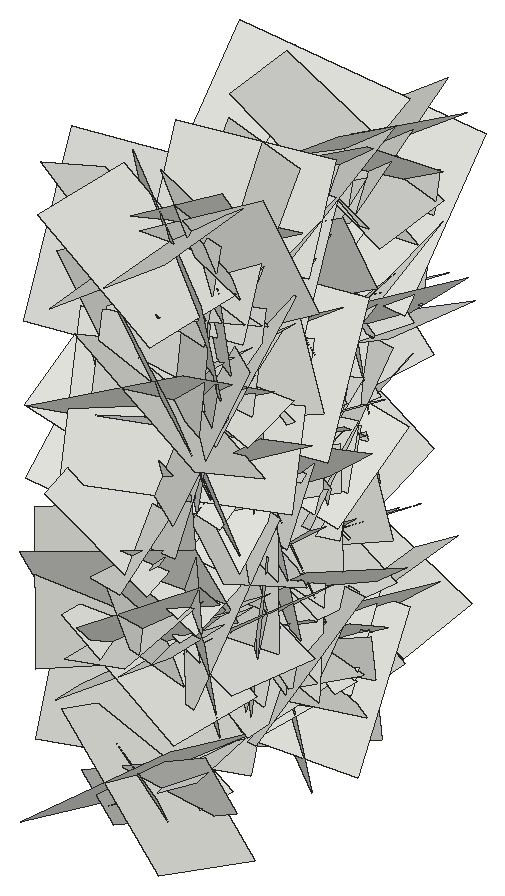
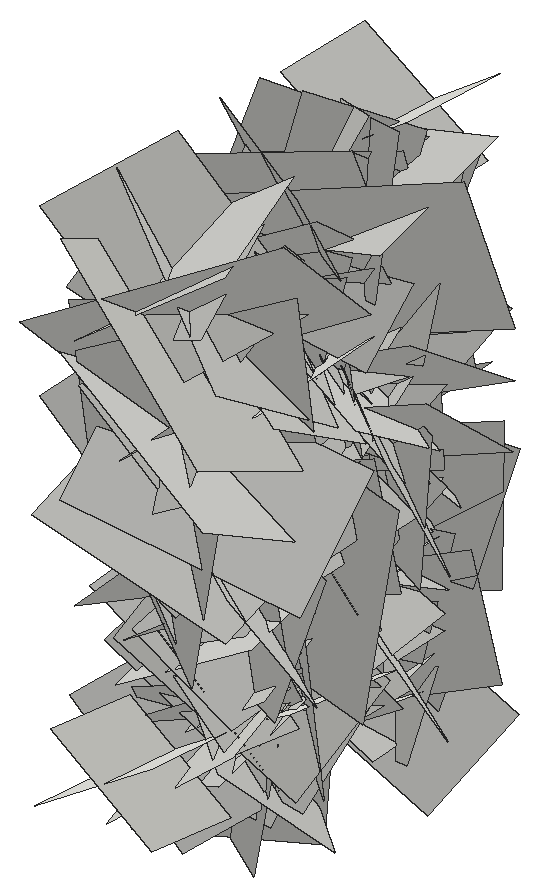
# SketchUp Ruby script. Lengths in inches.
U = 1.inch
M = Sketchup.active_model
def pt(a) = Geom::Point3d.new(a.map { |v| v * U })
def face(e, loops, mat)
  f = e.add_face(loops[0].map { |a| pt(a) })
  loops[1..].each { |l| e.add_face(l.map { |a| pt(a) }).erase! }
  f.material = f.back_material = mat if mat
  f
end
# faces: each face lists its corners as indices into pts; further lists are holes
def faces(e, pts, list, mat = nil) = list.each { |f| face(e, (f[0].is_a?(Array) ? f : [f]).map { |l| l.map { |i| pts[i] } }, mat) }
# xy, xz, yz: faces in a plane at the given z, y or x. An outline is a flat list of corners, or four numbers for a rectangle; further outlines are holes
def ring(l) = l.size == 4 ? [[l[0], l[1]], [l[2], l[1]], [l[2], l[3]], [l[0], l[3]]] : l.each_slice(2).to_a
def flat(e, list, mat, &to3) = list.each { |f| face(e, (f[0].is_a?(Array) ? f : [f]).map { |l| ring(l).map { |u, v| to3.(u, v) } }, mat) }
def xy(e, z, list, mat = nil) = flat(e, list, mat) { |x, y| [x, y, z] }
def xz(e, y, list, mat = nil) = flat(e, list, mat) { |x, z| [x, y, z] }
def yz(e, x, list, mat = nil) = flat(e, list, mat) { |y, z| [x, y, z] }
def lines(e, pts, list) = list.each { |a, b| e.add_line(pt(pts[a]), pt(pts[b])) }
# prism: a flat outline (further loops are holes) pulled along v
def prism(e, loops, v, mat = nil)
  f = face(e, loops, mat); d = Geom::Vector3d.new(v.map { |x| x * U })
  f.pushpull(f.normal.samedirection?(d) ? d.length : -d.length)
end
def box(e, o, s, mat = nil) = prism(e, [[o, [o[0] + s[0], o[1], o[2]], [o[0] + s[0], o[1] + s[1], o[2]], [o[0], o[1] + s[1], o[2]]]], [0, 0, s[2]], mat)
def at(x, y, z, deg = 0) = Geom::Transformation.translation(pt([x, y, z])) * Geom::Transformation.rotation(ORIGIN, Z_AXIS, deg.degrees)
def axes(o, x, y, z) = Geom::Transformation.new([*x, 0, *y, 0, *z, 0, *pt(o).to_a, 1])
def part(name) = M.definitions.add(name)
# library, detail: a bought-in or finely detailed component or shape, given as its bounding box
def library(name, o, s) = part(name).tap { |d| box(d.entities, o, s) }
def detail(e, o, s) = box(e.add_group.entities, o, s)
def put(e, d, t, mat = nil) = e.add_instance(d, t).tap { |i| i.material = mat if mat }
def group(e, t, mat = nil) = e.add_group.tap { |g| g.transformation = t; g.material = mat if mat }.entities
root = M.entities
c1 = part("Component\#6")
p = [[0.01,0,0],[0,3.24,4.54],[4.32,3.24,4.54],[4.33,0,0]]
faces(c1.entities,p,[[0,1,2,3]])
put(root,c1,axes([18.5,190.14,35.27],[-0.30668,1.10496,-0.445],[-0.14325,-0.48543,-1.11748],[-1.25452,-0.21469,0.23639]))
put(root,c1,axes([18.5,186.51,25.44],[0.00901,-0.3677,1.34811],[-0.26845,1.32541,0.3631],[-1.45667,-0.24653,-0.05858]))
put(root,c1,axes([18.5,188.1875,39.24],[-0.00053,-0.50504,-1.25708],[-0.1621,-1.24903,0.50186],[-1.42684,0.14209,-0.05655]))
put(root,c1,axes([18.5,180.73,30.67],[-0.05707,0.69485,1.12415],[0.04583,1.1254,-0.69356],[-1.4001,0.00851,-0.06852]))
put(root,c1,axes([18.5,188.72,38.18],[-0.108,1.17484,0.54266],[0.09899,0.5496,-1.17232],[-1.36819,-0.05298,-0.12766]))
put(root,c1,axes([18.5,187.26,33.24],[-0.066,-0.95024,-0.64083],[-0.19237,-0.6255,0.94515],[-1.19957,0.15259,-0.11631]))
put(root,c1,axes([18.5,181.61,25.33],[0.14764,0.72138,1.18272],[-0.09804,1.19088,-0.71546],[-1.46521,-0.007,0.16705]))
put(root,c1,axes([18.5,184.99,36.41],[-0.13687,-0.99381,0.45239],[-0.15227,0.46704,0.985],[-1.14738,0.05657,-0.18469]))
put(root,c1,axes([18.5,190.5,33.59],[-0.11278,1.05886,-0.21225],[-0.21462,-0.22906,-1.04119],[-1.12442,-0.06248,0.22002]))
put(root,c1,axes([18.5,187.29,32.09],[0.03087,-0.89426,-0.74249],[-0.26998,-0.72958,0.86873],[-1.20212,0.14089,-0.21417]))
put(root,c1,axes([18.5,186.91,28.91],[0.08475,0.77289,1.06783],[-0.0494,1.07079,-0.77154],[-1.39641,0.00903,0.0921]))
put(root,c1,axes([18.5,188.57,34.3],[0.02784,1.05016,0.5271],[-0.1514,0.52617,-1.0412],[-1.23628,-0.04079,0.13938]))
put(root,c1,axes([18.5,194.96,38.36],[0.08597,-0.96025,-0.92678],[0.03419,-0.92681,0.9631],[-1.41421,-0.08078,-0.03305]))
put(root,c1,axes([18.5,185.59,36.56],[-0.07365,1.00309,0.56692],[-0.00038,0.56794,-1.00493],[-1.22135,-0.06067,-0.03387]))
put(root,c1,axes([18.5,190.1,29],[-0.15352,-0.05709,1.12322],[0.06907,1.13017,0.06585],[-1.19015,0.07295,-0.14107]))
put(root,c1,axes([18.5,182.88,33.98],[-0.05541,0.90127,0.55592],[-0.17138,0.54328,-0.89597],[-1.1093,-0.12895,0.11065]))
put(root,c1,axes([18.5,181.98,27.65],[-0.03848,-0.07343,1.06513],[-0.13392,1.05855,0.06867],[-1.12376,-0.12364,-0.04466]))
put(root,c1,axes([14.53,188.74,27.6],[-0.13014,-0.45431,-0.37588],[-0.00674,-0.3829,0.46487],[0.62498,-0.09873,-0.07326]))
put(root,c1,axes([18.5,192.86,38.11],[-0.10772,-0.0541,-1.0459],[-0.04447,-1.04976,0.05837],[-1.10925,0.04734,0.09923]))
put(root,c1,axes([18.5,187.65,25.55],[-0.14301,-0.32766,0.90945],[-0.11586,0.91755,0.31436],[-1.01811,-0.05839,-0.16352]))
put(root,c1,axes([14.53,191.07,24.72],[-0.08022,-0.60182,-0.03468],[-0.03515,-0.03074,0.60586],[0.63802,-0.07736,0.02902]))
put(root,c1,axes([18.5,189.26,31.29],[-0.07003,-0.18149,-1.00879],[-0.05402,-1.00905,0.18487],[-1.08514,0.06195,0.0559]))
put(root,c1,axes([18.5,184.16,23.6],[-0.00632,0.19994,1.20323],[0.15077,1.19515,-0.1979],[-1.28409,0.13934,-0.02916]))
put(root,c1,axes([14.53,183.51,30.36],[-0.10644,-0.42009,-0.4575],[0.01901,-0.46521,0.42323],[0.65811,-0.0545,-0.08622]))
put(root,c1,axes([14.53,191.45,35.51],[-0.13227,0.51495,-0.41011],[-0.00116,-0.41758,-0.52399],[0.6978,0.09692,-0.07861]))
put(root,c1,axes([18.5,186.92,28.87],[-0.11772,1.08189,-0.3436],[0.18933,-0.32428,-1.0788],[-1.18826,-0.15885,-0.13785]))
put(root,c1,axes([18.5,185.29,39.56],[-0.11827,0.82487,-0.51088],[-0.03346,-0.51706,-0.82795],[-1.02793,-0.07808,0.08573]))
put(root,c1,axes([14.53,188.83,29.07],[-0.04972,0.59189,0.16701],[-0.02122,0.16593,-0.59371],[0.65156,0.05057,-0.00659]))
put(root,c1,axes([18.5,190.19,31.82],[-0.07854,-1.04848,0.11995],[0.05802,0.11627,1.05008],[-1.11713,0.07975,0.0461]))
put(root,c1,axes([14.53,186.02,29.02],[-0.12909,0.32312,-0.64935],[-0.06195,-0.66067,-0.31779],[0.76632,0.00102,-0.13508]))
put(root,c1,axes([18.5,185.55,26.35],[-0.05433,-0.24183,-1.04679],[0.06418,-1.04696,0.23891],[-1.13701,-0.04754,0.0635]))
put(root,c1,axes([18.5,185.63,37.94],[0.10296,1.07287,0.66666],[0.13207,0.65722,-1.07584],[-1.33238,0.14805,-0.05512]))
put(root,c1,axes([18.5,189.07,22.99],[-0.09993,-0.91741,-0.05408],[-0.10319,-0.04408,0.91762],[-0.96866,0.09934,-0.09218]))
put(root,c1,axes([14.53,193.29,29.97],[0.02765,-0.60791,0.13872],[-0.08921,0.13414,0.60366],[0.6549,0.04394,0.07638]))
put(root,c1,axes([14.53,188.93,38.32],[-0.06934,0.59373,0.25],[0.00198,0.25145,-0.59671],[0.68287,0.05956,0.02711]))
put(root,c1,axes([14.53,179.78,31.84],[-0.01485,0.68647,0.23212],[-0.1576,0.2245,-0.67291],[0.75179,0.06062,-0.13648]))
put(root,c1,axes([18.5,184.85,32.98],[0.15473,1.07562,-0.16592],[-0.16403,-0.14519,-1.07739],[-1.14193,0.1666,0.13228]))
put(root,c1,axes([18.5,181.64,30.57],[-0.02444,0.48831,-0.77146],[-0.19424,-0.75848,-0.47462],[-0.9481,0.1428,0.11713]))
put(root,c1,axes([18.5,182.41,31.86],[0.21699,-0.67676,1.03332],[-0.0082,1.04669,0.68705],[-1.3093,-0.11872,0.16695]))
put(root,c1,axes([14.53,185.35,37.93],[-0.06077,0.5182,0.40006],[0.00909,0.40215,-0.51968],[0.69387,0.04012,0.04185]))
put(root,c1,axes([14.53,183.4375,30.23],[-0.10865,-0.24445,0.66529],[0.00738,0.67183,0.24793],[0.75127,-0.04195,0.09378]))
put(root,c1,axes([14.53,183.98,26.9],[-0.15473,-0.64925,-0.29626],[0.07231,-0.3137,0.65387],[0.75301,-0.10329,-0.12366]))
put(root,c1,axes([14.53,188.41,35.3125],[0.03073,0.48255,0.4704],[-0.10717,0.46862,-0.47449],[0.70624,0.05011,-0.09248]))
put(root,c1,axes([18.5,187.18,35.87],[0.21905,1.32848,-0.23139],[0.18572,-0.25856,-1.32798],[-1.41727,0.17144,-0.20979]))
put(root,c1,axes([18.5,185.4,30.76],[0.02152,-0.00963,-1.2106],[0.23963,-1.18945,0.01326],[-1.26071,-0.22625,-0.01814]))
put(root,c1,axes([14.53,183.74,37.84],[0.08456,-0.37494,0.46177],[-0.03825,0.46199,0.38136],[0.62935,0.07846,-0.03886]))
put(root,c1,axes([14.53,188.62,32.29],[-0.0866,-0.74743,0.19758],[-0.06186,0.20408,0.74787],[0.81715,-0.06376,0.07755]))
put(root,c1,axes([14.53,184.65,28.76],[0.04824,-0.62434,-0.28052],[-0.09786,-0.28417,0.61748],[0.7189,0.00321,0.10288]))
put(root,c1,axes([18.5,186.48,30.64],[-0.03295,0.70699,0.47041],[-0.18441,0.45544,-0.69599],[-0.88105,-0.12176,0.12808]))
put(root,c1,axes([18.5,180.55,24.45],[-0.04702,0.95483,-0.28451],[0.08229,-0.28062,-0.95386],[-1.05288,-0.06457,-0.06184]))
put(root,c1,axes([18.5,184.8,33.37],[-0.19651,0.19461,-0.78555],[0.01158,-0.80522,-0.20206],[-0.85778,-0.05545,0.17724]))
put(root,c1,axes([18.5,181.12,36.49],[0.0887,0.85058,-0.45713],[-0.14057,-0.44437,-0.85112],[-1.01388,0.13603,0.07801]))
put(root,c1,axes([14.53,182.11,23.57],[-0.01533,0.32032,-0.55846],[0.07998,-0.55391,-0.31966],[0.67773,0.07262,0.02509]))
put(root,c1,axes([14.53,186.27,36.66],[-0.23271,0.08267,-1.0169],[-0.17131,-1.02986,-0.04883],[1.06781,-0.14721,-0.22945]))
put(root,c1,axes([14.53,181.88,29.24],[0.0732,0.47057,-0.46808],[-0.06498,-0.46407,-0.47558],[0.70054,-0.09222,0.00479]))
put(root,c1,axes([14.53,188.01,25.87],[-0.18323,0.88768,-0.1275],[-0.06793,-0.14175,-0.89995],[0.94816,0.16139,-0.08912]))
put(root,c1,axes([18.5,186.85,26],[-0.04759,0.74401,-0.43208],[-0.09551,-0.43435,-0.73856],[-0.90698,0.0067,0.10045]))
put(root,c1,axes([18.5,182.62,33.52],[0.16113,0.63843,0.91206],[0.00988,0.91976,-0.64538],[-1.18006,0.09488,0.11913]))
put(root,c1,axes([14.53,188.3,31.13],[-0.1103,-0.11339,-0.88165],[-0.13763,-0.87621,0.12802],[0.93214,-0.14279,-0.08543]))
put(root,c1,axes([18.5,182.86,27.86],[-0.00866,0.87216,-0.09866],[-0.12421,-0.09886,-0.86427],[-0.92206,0.00513,0.11735]))
put(root,c1,axes([14.53,188.48,31.6],[0.00806,0.51701,-0.38199],[0.06142,-0.38101,-0.51453],[0.67861,0.02834,0.0511]))
put(root,c1,axes([14.53,189.49,31],[-0.19159,0.03614,-0.77666],[0.1449,-0.78347,-0.06827],[0.81131,0.14846,-0.17121]))
put(root,c1,axes([18.5,186.8,27.07],[0.11611,-1.02809,0.5245],[0.14127,0.5346,1.02006],[-1.21522,-0.03608,0.16869]))
put(root,c1,axes([14.53,181.75,22.9],[0.07496,0.59984,0.04506],[0.05269,0.03939,-0.60235],[0.63545,-0.07402,0.04463]))
put(root,c1,axes([18.5,190.89,25.45],[0.07637,-0.93381,0.1535],[-0.06656,0.14888,0.93522],[-1.00091,-0.08115,-0.05048]))
put(root,c1,axes([18.5,189.24,21.76],[-0.15995,-0.688,0.38857],[0.02017,0.39231,0.70202],[-0.83731,0.14088,-0.05731]))
put(root,c1,axes([14.53,186.9,33.68],[-0.12726,-0.80704,-0.07778],[0.05104,-0.08559,0.81372],[0.85791,-0.11462,-0.05995]))
put(root,c1,axes([14.53,183.3,35.54],[0.06853,-0.0517,0.64839],[0.02911,0.65122,0.04919],[0.68886,-0.02238,-0.06659]))
put(root,c1,axes([18.5,182.91,34.72],[0.14912,-0.41506,0.98502],[0.044,0.99488,0.41329],[-1.13217,-0.016,0.1458]))
put(root,c1,axes([18.5,191.48,24.4],[0.24044,-0.84726,-0.84182],[0.11443,-0.83882,0.87332],[-1.26085,-0.2377,-0.08127]))
put(root,c1,axes([14.53,194.3125,23.26],[-0.02367,-0.75059,-0.08188],[0.02978,-0.08269,0.75031],[0.79979,-0.01914,-0.03036]))
put(root,c1,axes([18.5,189.58,22.99],[0.08755,-0.94666,0.34405],[0.04779,0.34833,0.94763],[-1.06661,-0.0621,0.0707]))
put(root,c1,axes([18.5,183.5625,38.07],[-0.03427,-0.86867,-0.02883],[0.01016,-0.0292,0.8692],[-0.92124,0.03199,0.01066]))
put(root,c1,axes([14.53,186.98,23.44],[-0.07046,0.41434,0.63319],[0.10971,0.63463,-0.40442],[0.79457,-0.05088,0.11199]))
put(root,c1,axes([18.5,186.99,20.26],[-0.04681,-0.17583,0.86867],[0.05724,0.86759,0.17835],[-0.93771,0.06173,-0.03248]))
put(root,c1,axes([14.53,182.78,23.92],[-0.06221,-0.24398,0.83625],[-0.07047,0.83695,0.23952],[0.92069,0.04758,0.07484]))
put(root,c1,axes([18.5,187.32,34.27],[-0.05201,-0.4187,0.7383],[0.02779,0.73844,0.42051],[-0.89926,0.04704,-0.0297]))
put(root,c1,axes([14.53,187.84,31.26],[0.01205,0.8882,0.30464],[-0.22592,0.29915,-0.86424],[0.96935,0.05868,-0.20521]))
put(root,c1,axes([14.53,187.61,26.86],[-0.07932,-0.16974,-0.83453],[-0.0041,-0.83766,0.17072],[0.9027,-0.01872,-0.07255]))
put(root,c1,axes([14.53,184.84,39.1],[0.02023,-0.20369,-0.6632],[0.11732,-0.65406,0.20407],[0.72599,0.11137,-0.0145]))
put(root,c1,axes([18.5,180.54,27.52],[-0.00647,0.86334,-0.00303],[0.00368,-0.003,-0.86336],[-0.91514,-0.00612,-0.00345]))
put(root,c1,axes([18.5,189.53,40.3125],[0.07096,0.70634,-0.4758],[-0.12627,-0.46481,-0.70678],[-0.89387,0.12173,0.06207]))
put(root,c1,axes([18.5,192.58,32.17],[-0.11188,-0.86522,-0.03173],[0.14554,-0.04829,0.85998],[-0.90613,0.09907,0.14204]))
put(root,c1,axes([18.5,185.86,28.71],[0.06844,0.29244,0.76285],[-0.17475,0.75415,-0.27515],[-0.84819,-0.13178,0.11824]))
put(root,c1,axes([14.53,188.23,41.22],[-0.26749,1.02168,-0.17372],[0.00845,-0.17688,-1.05183],[1.0985,0.25014,-0.03421]))
put(root,c1,axes([18.5,187.08,35.11],[0.23629,-0.52338,-1.02054],[0.13084,-1.02265,0.55142],[-1.20867,-0.21302,-0.13982]))
put(root,c1,axes([14.53,187.74,23.43],[-0.08523,-0.9506,0.05636],[-0.09187,0.06363,0.94959],[1.00521,-0.07479,0.09156]))
put(root,c1,axes([14.53,184.52,38.07],[-0.06477,0.36641,0.7198],[0.11209,0.71927,-0.35717],[0.84878,-0.06703,0.10209]))
put(root,c1,axes([14.53,184.92,37.05],[0.01613,-0.13323,-0.78421],[0.01491,-0.78419,0.1335],[0.84304,0.01642,0.01265]))
put(root,c1,axes([18.5,184.92,37.05],[-0.01613,-0.13323,-0.78421],[-0.01491,-0.78419,0.1335],[-0.84304,0.01642,0.01265]))
put(root,c1,axes([18.5,184.52,38.07],[0.06477,0.36641,0.7198],[-0.11209,0.71927,-0.35717],[-0.84878,-0.06703,0.10209]))
put(root,c1,axes([18.5,187.74,23.43],[0.08523,-0.9506,0.05636],[0.09187,0.06363,0.94959],[-1.00521,-0.07479,0.09156]))
put(root,c1,axes([14.53,187.08,35.11],[-0.23629,-0.52338,-1.02054],[-0.13084,-1.02265,0.55142],[1.20867,-0.21302,-0.13982]))
put(root,c1,axes([18.5,188.23,41.22],[0.26749,1.02168,-0.17372],[-0.00845,-0.17688,-1.05183],[-1.0985,0.25014,-0.03421]))
put(root,c1,axes([14.53,185.86,28.71],[-0.06844,0.29244,0.76285],[0.17475,0.75415,-0.27515],[0.84819,-0.13178,0.11824]))
put(root,c1,axes([14.53,192.58,32.17],[0.11188,-0.86522,-0.03173],[-0.14554,-0.04829,0.85998],[0.90613,0.09907,0.14204]))
put(root,c1,axes([14.53,189.53,40.3125],[-0.07096,0.70634,-0.4758],[0.12627,-0.46481,-0.70678],[0.89387,0.12173,0.06207]))
put(root,c1,axes([14.53,180.54,27.52],[0.00647,0.86334,-0.00303],[-0.00368,-0.003,-0.86336],[0.91514,-0.00612,-0.00345]))
put(root,c1,axes([18.5,184.84,39.1],[-0.02023,-0.20369,-0.6632],[-0.11732,-0.65406,0.20407],[-0.72599,0.11137,-0.0145]))
put(root,c1,axes([18.5,187.61,26.86],[0.07932,-0.16974,-0.83453],[0.0041,-0.83766,0.17072],[-0.9027,-0.01872,-0.07255]))
put(root,c1,axes([18.5,187.84,31.26],[-0.01205,0.8882,0.30464],[0.22592,0.29915,-0.86424],[-0.96935,0.05868,-0.20521]))
put(root,c1,axes([14.53,187.32,34.27],[0.05201,-0.4187,0.7383],[-0.02779,0.73844,0.42051],[0.89926,0.04704,-0.0297]))
put(root,c1,axes([18.5,182.78,23.92],[0.06221,-0.24398,0.83625],[0.07047,0.83695,0.23952],[-0.92069,0.04758,0.07484]))
put(root,c1,axes([14.53,186.99,20.26],[0.04681,-0.17583,0.86867],[-0.05724,0.86759,0.17835],[0.93771,0.06173,-0.03248]))
put(root,c1,axes([18.5,186.98,23.44],[0.07046,0.41434,0.63319],[-0.10971,0.63463,-0.40442],[-0.79457,-0.05088,0.11199]))
put(root,c1,axes([14.53,183.5625,38.07],[0.03427,-0.86867,-0.02883],[-0.01016,-0.0292,0.8692],[0.92124,0.03199,0.01066]))
put(root,c1,axes([14.53,189.58,22.99],[-0.08755,-0.94666,0.34405],[-0.04779,0.34833,0.94763],[1.06661,-0.0621,0.0707]))
put(root,c1,axes([18.5,194.3125,23.26],[0.02367,-0.75059,-0.08188],[-0.02978,-0.08269,0.75031],[-0.79979,-0.01914,-0.03036]))
put(root,c1,axes([14.53,191.48,24.4],[-0.24044,-0.84726,-0.84182],[-0.11443,-0.83882,0.87332],[1.26085,-0.2377,-0.08127]))
put(root,c1,axes([14.53,182.91,34.72],[-0.14912,-0.41506,0.98502],[-0.044,0.99488,0.41329],[1.13217,-0.016,0.1458]))
put(root,c1,axes([18.5,183.3,35.54],[-0.06853,-0.0517,0.64839],[-0.02911,0.65122,0.04919],[-0.68886,-0.02238,-0.06659]))
put(root,c1,axes([18.5,186.9,33.68],[0.12726,-0.80704,-0.07778],[-0.05104,-0.08559,0.81372],[-0.85791,-0.11462,-0.05995]))
put(root,c1,axes([14.53,189.24,21.76],[0.15995,-0.688,0.38857],[-0.02017,0.39231,0.70202],[0.83731,0.14088,-0.05731]))
put(root,c1,axes([14.53,190.89,25.45],[-0.07637,-0.93381,0.1535],[0.06656,0.14888,0.93522],[1.00091,-0.08115,-0.05048]))
put(root,c1,axes([18.5,181.75,22.9],[-0.07496,0.59984,0.04506],[-0.05269,0.03939,-0.60235],[-0.63545,-0.07402,0.04463]))
put(root,c1,axes([14.53,186.8,27.07],[-0.11611,-1.02809,0.5245],[-0.14127,0.5346,1.02006],[1.21522,-0.03608,0.16869]))
put(root,c1,axes([18.5,189.49,31],[0.19159,0.03614,-0.77666],[-0.1449,-0.78347,-0.06827],[-0.81131,0.14846,-0.17121]))
put(root,c1,axes([18.5,188.48,31.6],[-0.00806,0.51701,-0.38199],[-0.06142,-0.38101,-0.51453],[-0.67861,0.02834,0.0511]))
put(root,c1,axes([14.53,182.86,27.86],[0.00866,0.87216,-0.09866],[0.12421,-0.09886,-0.86427],[0.92206,0.00513,0.11735]))
put(root,c1,axes([18.5,188.3,31.13],[0.1103,-0.11339,-0.88165],[0.13763,-0.87621,0.12802],[-0.93214,-0.14279,-0.08543]))
put(root,c1,axes([14.53,182.62,33.52],[-0.16113,0.63843,0.91206],[-0.00988,0.91976,-0.64538],[1.18006,0.09488,0.11913]))
put(root,c1,axes([14.53,186.85,26],[0.04759,0.74401,-0.43208],[0.09551,-0.43435,-0.73856],[0.90698,0.0067,0.10045]))
put(root,c1,axes([18.5,188.01,25.87],[0.18323,0.88768,-0.1275],[0.06793,-0.14175,-0.89995],[-0.94816,0.16139,-0.08912]))
put(root,c1,axes([18.5,181.88,29.24],[-0.0732,0.47057,-0.46808],[0.06498,-0.46407,-0.47558],[-0.70054,-0.09222,0.00479]))
put(root,c1,axes([18.5,186.27,36.66],[0.23271,0.08267,-1.0169],[0.17131,-1.02986,-0.04883],[-1.06781,-0.14721,-0.22945]))
put(root,c1,axes([18.5,182.11,23.57],[0.01533,0.32032,-0.55846],[-0.07998,-0.55391,-0.31966],[-0.67773,0.07262,0.02509]))
put(root,c1,axes([14.53,181.12,36.49],[-0.0887,0.85058,-0.45713],[0.14057,-0.44437,-0.85112],[1.01388,0.13603,0.07801]))
put(root,c1,axes([14.53,184.8,33.37],[0.19651,0.19461,-0.78555],[-0.01158,-0.80522,-0.20206],[0.85778,-0.05545,0.17724]))
put(root,c1,axes([14.53,180.55,24.45],[0.04702,0.95483,-0.28451],[-0.08229,-0.28062,-0.95386],[1.05288,-0.06457,-0.06184]))
put(root,c1,axes([14.53,186.48,30.64],[0.03295,0.70699,0.47041],[0.18441,0.45544,-0.69599],[0.88105,-0.12176,0.12808]))
put(root,c1,axes([18.5,184.65,28.76],[-0.04824,-0.62434,-0.28052],[0.09786,-0.28417,0.61748],[-0.7189,0.00321,0.10288]))
put(root,c1,axes([18.5,188.62,32.29],[0.0866,-0.74743,0.19758],[0.06186,0.20408,0.74787],[-0.81715,-0.06376,0.07755]))
put(root,c1,axes([18.5,183.74,37.84],[-0.08456,-0.37494,0.46177],[0.03825,0.46199,0.38136],[-0.62935,0.07846,-0.03886]))
